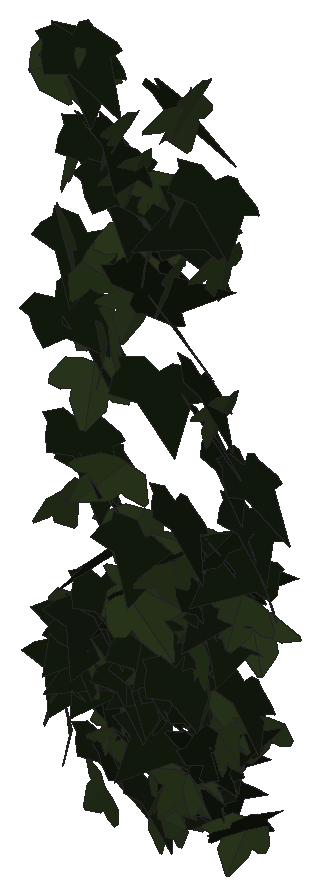
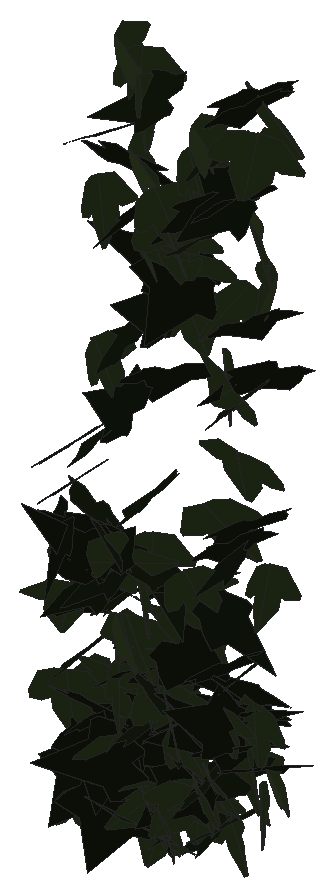
# SketchUp Ruby script. Lengths in inches.
U = 1.inch
M = Sketchup.active_model
def pt(a) = Geom::Point3d.new(a.map { |v| v * U })
def face(e, loops, mat)
  f = e.add_face(loops[0].map { |a| pt(a) })
  loops[1..].each { |l| e.add_face(l.map { |a| pt(a) }).erase! }
  f.material = f.back_material = mat if mat
  f
end
# faces: each face lists its corners as indices into pts; further lists are holes
def faces(e, pts, list, mat = nil) = list.each { |f| face(e, (f[0].is_a?(Array) ? f : [f]).map { |l| l.map { |i| pts[i] } }, mat) }
# xy, xz, yz: faces in a plane at the given z, y or x. An outline is a flat list of corners, or four numbers for a rectangle; further outlines are holes
def ring(l) = l.size == 4 ? [[l[0], l[1]], [l[2], l[1]], [l[2], l[3]], [l[0], l[3]]] : l.each_slice(2).to_a
def flat(e, list, mat, &to3) = list.each { |f| face(e, (f[0].is_a?(Array) ? f : [f]).map { |l| ring(l).map { |u, v| to3.(u, v) } }, mat) }
def xy(e, z, list, mat = nil) = flat(e, list, mat) { |x, y| [x, y, z] }
def xz(e, y, list, mat = nil) = flat(e, list, mat) { |x, z| [x, y, z] }
def yz(e, x, list, mat = nil) = flat(e, list, mat) { |y, z| [x, y, z] }
def lines(e, pts, list) = list.each { |a, b| e.add_line(pt(pts[a]), pt(pts[b])) }
# prism: a flat outline (further loops are holes) pulled along v
def prism(e, loops, v, mat = nil)
  f = face(e, loops, mat); d = Geom::Vector3d.new(v.map { |x| x * U })
  f.pushpull(f.normal.samedirection?(d) ? d.length : -d.length)
end
def box(e, o, s, mat = nil) = prism(e, [[o, [o[0] + s[0], o[1], o[2]], [o[0] + s[0], o[1] + s[1], o[2]], [o[0], o[1] + s[1], o[2]]]], [0, 0, s[2]], mat)
def at(x, y, z, deg = 0) = Geom::Transformation.translation(pt([x, y, z])) * Geom::Transformation.rotation(ORIGIN, Z_AXIS, deg.degrees)
def axes(o, x, y, z) = Geom::Transformation.new([*x, 0, *y, 0, *z, 0, *pt(o).to_a, 1])
def part(name) = M.definitions.add(name)
# library, detail: a bought-in or finely detailed component or shape, given as its bounding box
def library(name, o, s) = part(name).tap { |d| box(d.entities, o, s) }
def detail(e, o, s) = box(e.add_group.entities, o, s)
def put(e, d, t, mat = nil) = e.add_instance(d, t).tap { |i| i.material = mat if mat }
def group(e, t, mat = nil) = e.add_group.tap { |g| g.transformation = t; g.material = mat if mat }.entities
root = M.entities
M.materials.add("1026 AP 7946 SUNNY SIDE UP").color = [254, 231, 186]
M.materials.add("efeu1").color = [18, 25, 13]
M.materials.add("efeu2").color = [43, 57, 29]
c1 = part("ivyleaf_10")
p = [[0,0.5,-0.03],[-0.0625,2.02,-0.43],[-0.19,2.01,-0.46],[-0.54,1.05,-0.29],[-0.52,0.625,-0.18],[-0.83,0.76,-0.28],
  [-1.16,0.64,-0.33],[-1.15,0.33,-0.24],[-0.77,-0.39,0.02],[-0.3,-0.51,0.16],[0.04,-0.48,0.23],[-0.02,2.01,-0.4375],
  [-0.06,2.01,-0.43],[0.04,-0.49,0.23],[0.67,-0.49,0.14],[1.38,0.36,-0.2],[1.375,0.51,-0.24],[0.81,0.65,-0.19],
  [0.62,0.59,-0.15],[0.6,1.09,-0.28],[0.5,1.23,-0.31]]
faces(c1.entities,p,[[0,1,2,3,4,5,6,7,8,9,10],[11,12,0,13,14,15,16,17,18,19,20]],"efeu2")
c2 = part("ivyleaf_9")
p = [[1.54,2.16,1.25],[1.36,2.04,1.19],[-0.21,0.99,0.68],[-0.71,1.11,0.82],[-0.85,0.86,0.67],[-0.8,0.17,0.21],
  [-0.9,-0.01,0.1],[-0.67,-0.16,-0.02],[-0.08,-0.08,-0.05],[-0.03,-0.6,-0.4],[0.65,-0.88,-0.66],[0.83,-0.6,-0.49],
  [1.29,-0.42,-0.43],[1.8125,-0.07,-0.26],[1.21,0.44,0.15]]
faces(c2.entities,p,[[0,1,2,3,4,5,6,7,8,9,10,11,12,13,14]],"efeu1")
put(root,c1,axes([125.9,212.72,288.875],[0.27031,-0.30835,-0.02636],[-0.00295,0.02623,-0.36336],[0.48629,0.17156,0.01245]),"1026 AP 7946 SUNNY SIDE UP")
put(root,c1,axes([125.88,212.42,280.78],[0.18915,-0.27946,0.07883],[0.04242,-0.07342,-0.31384],[0.45429,0.12321,-0.00352]),"1026 AP 7946 SUNNY SIDE UP")
put(root,c1,axes([125.91,212.75,290.12],[-0.49029,-0.16213,-0.04358],[0.07501,-0.00225,-0.36123],[0.25219,-0.31453,0.02272]),"1026 AP 7946 SUNNY SIDE UP")
put(root,c1,axes([125.86,212.73,281.77],[0.4363,-0.17051,-0.03418],[0.03314,0.09342,-0.32184],[0.27083,0.26325,0.09445]),"1026 AP 7946 SUNNY SIDE UP")
put(root,c1,axes([125.91,212.43,283.64],[-0.11924,-0.2929,-0.13998],[0.08747,0.12391,-0.31023],[0.499,-0.09171,0.02093]),"1026 AP 7946 SUNNY SIDE UP")
put(root,c1,axes([125.6,212.43,290.15],[0.31014,-0.19111,-0.25299],[0.32846,-0.13247,0.2795],[-0.36084,-0.28483,0.03698]),"1026 AP 7946 SUNNY SIDE UP")
put(root,c2,axes([125.93,212.75,280.98],[-0.30569,-0.24857,0.06162],[0.05661,-0.10267,-0.31222],[0.39854,-0.17608,0.09162]),"1026 AP 7946 SUNNY SIDE UP")
put(root,c1,axes([126.25,212.53,280.91],[-0.19821,0.12164,0.30818],[-0.38939,0.16855,-0.17753],[-0.32434,-0.27669,0.0248]),"1026 AP 7946 SUNNY SIDE UP")
put(root,c1,axes([125.98,212.35,287.9375],[-0.27058,0.28491,-0.09651],[0.04338,-0.09437,-0.34254],[-0.47039,-0.17259,0.02392]),"1026 AP 7946 SUNNY SIDE UP")
put(root,c2,axes([126.01,212.8,287.54],[-0.20232,-0.3188,0.03575],[0.0034,-0.0402,-0.35397],[0.50455,-0.12757,0.01672]),"1026 AP 7946 SUNNY SIDE UP")
put(root,c1,axes([126.18,212.21,280.22],[0.12911,-0.18145,-0.26592],[-0.07081,0.25619,-0.19959],[0.48971,0.08488,0.04125]),"1026 AP 7946 SUNNY SIDE UP")
put(root,c2,axes([126.17,212.68,281.64],[-0.35105,-0.22264,0.09145],[-0.02769,-0.10742,-0.31927],[0.3766,-0.21543,0.06177]),"1026 AP 7946 SUNNY SIDE UP")
put(root,c2,axes([125.9375,212.77,284.62],[0.03499,-0.32884,-0.11313],[0.0607,0.10985,-0.33591],[0.54081,0.00894,0.04502]),"1026 AP 7946 SUNNY SIDE UP")
put(root,c2,axes([125.89,212.36,286.68],[0.12891,-0.22324,-0.27152],[0.08477,0.27461,-0.22182],[0.53491,0.01028,0.10059]),"1026 AP 7946 SUNNY SIDE UP")
put(root,c1,axes([126.13,212.74,285.45],[0.55471,-0.02774,0.05101],[0.07311,-0.03924,-0.36298],[0.05156,0.35409,-0.03412]),"1026 AP 7946 SUNNY SIDE UP")
put(root,c2,axes([126.08,212.84,286.34],[0.07413,-0.33284,0.0505],[0.00087,-0.05133,-0.34655],[0.52945,0.04669,-0.0065]),"1026 AP 7946 SUNNY SIDE UP")
put(root,c2,axes([126.16,212.62,290.58],[-0.08016,-0.35944,0.00458],[0.00034,-0.00658,-0.37404],[0.56528,-0.05097,0.00088]),"1026 AP 7946 SUNNY SIDE UP")
put(root,c2,axes([126.2,212.88,284.26],[-0.11359,-0.32153,-0.00731],[0.00034,0.00535,-0.33947],[0.50565,-0.07224,-0.00142]),"1026 AP 7946 SUNNY SIDE UP")
put(root,c2,axes([126.09,212.46,290.75],[0.05375,-0.31546,-0.17041],[0.04786,0.16637,-0.32292],[0.55673,0.01615,0.04421]),"1026 AP 7946 SUNNY SIDE UP")
put(root,c2,axes([126.13,212.76,284.125],[0.3525,-0.23972,-0.11649],[-0.14407,0.06698,-0.3371],[0.39011,0.24135,-0.01924]),"1026 AP 7946 SUNNY SIDE UP")
put(root,c1,axes([126.2,212.42,281.45],[-0.34069,0.13509,-0.19375],[0.16571,-0.17294,-0.25302],[-0.32532,-0.22956,0.07403]),"1026 AP 7946 SUNNY SIDE UP")
put(root,c2,axes([126.22,212.93,281.52],[0.07138,-0.00129,0.32422],[0.35069,0.22449,-0.03088],[-0.34918,0.2252,0.03526]),"1026 AP 7946 SUNNY SIDE UP")
put(root,c2,axes([126.42,212.77,281.08],[-0.31851,-0.23754,0.08271],[0.01533,-0.11223,-0.31217],[0.39466,-0.18735,0.07888]),"1026 AP 7946 SUNNY SIDE UP")
put(root,c2,axes([126.25,212.72,289.22],[-0.01907,-0.35238,-0.04597],[0.0006,0.04263,-0.36298],[0.55812,-0.01209,-0.00118]),"1026 AP 7946 SUNNY SIDE UP")
put(root,c2,axes([126.62,212.67,281.27],[-0.38905,-0.15491,0.14585],[-0.16155,-0.10298,-0.2998],[0.2888,-0.26629,0.02878]),"1026 AP 7946 SUNNY SIDE UP")
put(root,c2,axes([126.35,212.63,281.67],[-0.2732,-0.25599,-0.07802],[0.12245,0.03605,-0.31543],[0.40084,-0.18549,0.04318]),"1026 AP 7946 SUNNY SIDE UP")
put(root,c2,axes([126.2,212.74,289.29],[0.51186,-0.12067,-0.05066],[-0.0863,-0.00897,-0.35661],[0.18539,0.329,-0.02612]),"1026 AP 7946 SUNNY SIDE UP")
put(root,c2,axes([126.64,212.5625,283.01],[-0.20337,0.23142,-0.18939],[0.05782,-0.18793,-0.26954],[-0.46242,-0.12527,0.04959]),"1026 AP 7946 SUNNY SIDE UP")
put(root,c2,axes([126.13,212.58,280.71],[0.20887,-0.26076,0.11855],[0.15681,-0.07811,-0.29757],[0.42084,0.15852,0.05204]),"1026 AP 7946 SUNNY SIDE UP")
put(root,c2,axes([126.5,212.5625,281.96],[-0.44635,-0.14929,-0.08709],[0.13609,0.0146,-0.3292],[0.23217,-0.29558,0.02555]),"1026 AP 7946 SUNNY SIDE UP")
put(root,c2,axes([126.29,212.8125,282.09],[0.07857,-0.32043,0.03112],[0.00011,-0.0324,-0.33425],[0.50636,0.04973,-0.00475]),"1026 AP 7946 SUNNY SIDE UP")
put(root,c1,axes([126.5,212.82,281.64],[0.48968,-0.07394,-0.03517],[-0.05512,-0.00175,-0.3296],[0.11529,0.31324,-0.00821]),"1026 AP 7946 SUNNY SIDE UP")
put(root,c2,axes([126.37,212.72,282.35],[0.03697,-0.30768,-0.09831],[0.0408,0.09544,-0.31565],[0.50408,0.01484,0.03276]),"1026 AP 7946 SUNNY SIDE UP")
put(root,c2,axes([126.38,212.71,279.98],[0.08932,-0.30861,-0.02061],[0.0869,0.0284,-0.31726],[0.47828,0.05248,0.06149]),"1026 AP 7946 SUNNY SIDE UP")
put(root,c1,axes([126.78,212.48,284.31],[0.39586,0.12783,-0.19321],[-0.30675,-0.02334,-0.2852],[-0.18425,0.3135,0.0597]),"1026 AP 7946 SUNNY SIDE UP")
put(root,c1,axes([126.52,212.24,287.49],[-0.09273,-0.24523,-0.26318],[0.24366,0.21349,-0.24808],[0.49892,-0.14984,0.07225]),"1026 AP 7946 SUNNY SIDE UP")
put(root,c1,axes([126.34,212.68,286.35],[0.39385,-0.05844,0.25761],[0.36023,-0.10799,-0.26268],[0.18356,0.3373,-0.03723]),"1026 AP 7946 SUNNY SIDE UP")
put(root,c1,axes([126.92,212.05,279.6],[-0.30668,0.14917,0.22949],[-0.33738,0.07661,-0.24687],[-0.25091,-0.28534,0.05145]),"1026 AP 7946 SUNNY SIDE UP")
put(root,c1,axes([126.625,212.65,280.45],[0.35829,-0.19594,0.09833],[0.08114,-0.08731,-0.30845],[0.33375,0.23157,-0.03057]),"1026 AP 7946 SUNNY SIDE UP")
put(root,c1,axes([126.8,212.17,286.36],[0.20652,-0.26363,-0.20979],[-0.04754,0.20698,-0.29712],[0.5202,0.12358,0.05613]),"1026 AP 7946 SUNNY SIDE UP")
put(root,c2,axes([126.45,212.47,281.18],[0.29811,0.09709,0.24138],[0.34076,0.08864,-0.21848],[-0.20564,0.28762,-0.01212]),"1026 AP 7946 SUNNY SIDE UP")
put(root,c1,axes([126.73,212.81,280.33],[0.3077,-0.24861,0.03727],[0.04569,-0.02495,-0.32599],[0.3927,0.1977,0.00872]),"1026 AP 7946 SUNNY SIDE UP")
put(root,c1,axes([126.86,212.87,283.4375],[-0.27049,-0.24659,0.13294],[-0.00508,-0.15148,-0.30028],[0.43863,-0.15382,0.07851]),"1026 AP 7946 SUNNY SIDE UP")
put(root,c2,axes([126.59,212.62,279.84],[0.26914,-0.26132,-0.04178],[-0.04522,0.02786,-0.32153],[0.41301,0.17334,-0.00797]),"1026 AP 7946 SUNNY SIDE UP")
put(root,c1,axes([126.95,212.65,280.22],[-0.41449,-0.18507,0.01137],[0.00557,-0.02604,-0.33109],[0.29157,-0.26259,0.0225]),"1026 AP 7946 SUNNY SIDE UP")
put(root,c2,axes([126.67,212.51,288.95],[0.11307,-0.22963,-0.27403],[0.02992,0.27237,-0.2365],[0.55018,0.03238,0.06918]),"1026 AP 7946 SUNNY SIDE UP")
put(root,c2,axes([126.67,212.73,280.51],[0.19701,-0.29561,0.00896],[0.00684,-0.00942,-0.33081],[0.46505,0.12537,0.00107]),"1026 AP 7946 SUNNY SIDE UP")
put(root,c2,axes([127.07,212.78,282.39],[-0.0711,0.15814,-0.28677],[0.04928,-0.27849,-0.16933],[-0.50222,-0.04971,0.02398]),"1026 AP 7946 SUNNY SIDE UP")
put(root,c1,axes([126.98,212.48,289.76],[0.07132,-0.32502,0.13566],[0.00688,-0.1341,-0.33859],[0.55246,0.04363,-0.0133]),"1026 AP 7946 SUNNY SIDE UP")
put(root,c1,axes([127.23,212.54,282.59],[-0.39985,0.02202,0.20204],[-0.29352,-0.13008,-0.23522],[0.10009,-0.29353,0.11733]),"1026 AP 7946 SUNNY SIDE UP")
put(root,c2,axes([126.83,212.72,288.43],[-0.08218,-0.30684,0.16377],[0.05503,-0.16638,-0.3165],[0.54187,-0.02964,0.05698]),"1026 AP 7946 SUNNY SIDE UP")
put(root,c1,axes([127.05,212.8,281.08],[-0.12394,-0.27894,0.13465],[0.0106,-0.13806,-0.29656],[0.48533,-0.06822,0.04087]),"1026 AP 7946 SUNNY SIDE UP")
put(root,c2,axes([126.93,212.47,289.38],[-0.10267,-0.25655,0.24066],[0.04118,-0.24211,-0.26615],[0.54558,-0.03001,0.06538]),"1026 AP 7946 SUNNY SIDE UP")
put(root,c2,axes([127.01,212.65,281.26],[-0.12456,-0.30558,-0.05106],[0.04831,0.04135,-0.32437],[0.48393,-0.08278,0.01924]),"1026 AP 7946 SUNNY SIDE UP")
put(root,c1,axes([127.04,212.74,280.15],[-0.35078,-0.16321,-0.15919],[0.21561,0.07202,-0.2836],[0.27874,-0.2611,0.01904]),"1026 AP 7946 SUNNY SIDE UP")
put(root,c1,axes([127.21,212.35,289.25],[-0.06477,-0.36023,-0.00274],[0.01132,-0.00021,-0.37345],[0.56631,-0.04119,0.00715]),"1026 AP 7946 SUNNY SIDE UP")
put(root,c2,axes([127.09,212.7,283.28],[-0.201,-0.30566,0.04261],[0.00852,-0.04886,-0.34073],[0.4853,-0.12574,0.02363]),"1026 AP 7946 SUNNY SIDE UP")
put(root,c1,axes([127.25,212.4375,287.1875],[-0.2232,-0.30509,0.10051],[-0.00382,-0.10755,-0.34465],[0.50448,-0.1358,0.04186]),"1026 AP 7946 SUNNY SIDE UP")
put(root,c1,axes([127.08,212.57,287.96],[0.52468,0.11095,0.0094],[0.03089,-0.03233,-0.36045],[-0.17223,0.33222,-0.03603]),"1026 AP 7946 SUNNY SIDE UP")
put(root,c2,axes([126.99,212.62,280.34],[0.50426,-0.02227,-0.0261],[-0.04234,-0.02522,-0.33016],[0.03169,0.32069,-0.02588]),"1026 AP 7946 SUNNY SIDE UP")
put(root,c1,axes([127.375,212.65,288.32],[-0.51079,-0.08402,0.10248],[-0.12848,-0.07825,-0.34179],[0.16016,-0.33075,0.05266]),"1026 AP 7946 SUNNY SIDE UP")
put(root,c1,axes([127.25,212.8,281.48],[0.14073,-0.30596,-0.05661],[-0.00093,0.05521,-0.32773],[0.48831,0.08828,0.01569]),"1026 AP 7946 SUNNY SIDE UP")
put(root,c2,axes([127.11,212.63,287.72],[0.51596,0.0352,-0.11248],[-0.16844,-0.02599,-0.33984],[-0.06535,0.3449,-0.01208]),"1026 AP 7946 SUNNY SIDE UP")
put(root,c2,axes([127.15,212.8,281.21],[-0.1011,-0.30619,0.07614],[0.00569,-0.07792,-0.32218],[0.4959,-0.06153,0.01922]),"1026 AP 7946 SUNNY SIDE UP")
put(root,c2,axes([127.57,212.76,281.625],[-0.35,0.23567,-0.02127],[-0.00684,-0.03425,-0.33303],[-0.37212,-0.22103,0.02613]),"1026 AP 7946 SUNNY SIDE UP")
put(root,c1,axes([127.41,212.76,281.46],[-0.33834,-0.2305,0.07924],[-0.01901,-0.09416,-0.32063],[0.38226,-0.20869,0.05419]),"1026 AP 7946 SUNNY SIDE UP")
put(root,c2,axes([127.52,212.65,280.92],[-0.38418,0.18598,-0.08726],[0.09009,-0.06609,-0.31622],[-0.30917,-0.25036,0.01628]),"1026 AP 7946 SUNNY SIDE UP")
put(root,c1,axes([127.41,212.79,288.8125],[-0.24704,-0.29268,0.1131],[0.00476,-0.12609,-0.33749],[0.49242,-0.14561,0.06]),"1026 AP 7946 SUNNY SIDE UP")
put(root,c2,axes([127.56,212.76,281.42],[-0.48913,-0.08331,0.04318],[-0.05175,-0.04025,-0.33054],[0.13757,-0.31136,0.02919]),"1026 AP 7946 SUNNY SIDE UP")
put(root,c2,axes([127.23,212.61,279.62],[0.08962,-0.30503,0.04262],[0.02998,-0.04026,-0.3197],[0.48346,0.05904,0.01193]),"1026 AP 7946 SUNNY SIDE UP")
put(root,c2,axes([127.67,212.49,283.23],[-0.03751,0.31967,0.07441],[-0.07471,0.06648,-0.32707],[-0.50925,-0.0333,0.0425]),"1026 AP 7946 SUNNY SIDE UP")
put(root,c1,axes([127.38,212.54,288.19],[0.22506,-0.26703,0.19485],[0.16607,-0.15944,-0.31267],[0.48846,0.17724,0.01653]),"1026 AP 7946 SUNNY SIDE UP")
put(root,c2,axes([127.37,212.5625,281.82],[-0.15335,-0.29472,-0.10509],[0.07123,0.09059,-0.31896],[0.48433,-0.10664,0.01364]),"1026 AP 7946 SUNNY SIDE UP")
put(root,c1,axes([127.1875,212.37,282.39],[0.40212,0.09619,0.21799],[0.31879,0.05989,-0.28085],[-0.17714,0.32613,-0.01058]),"1026 AP 7946 SUNNY SIDE UP")
put(root,c1,axes([127.54,212.52,279.67],[0.15211,-0.29945,-0.02419],[0.02958,0.02888,-0.32285],[0.47117,0.09486,0.02808]),"1026 AP 7946 SUNNY SIDE UP")
put(root,c1,axes([127.59,212.78,279.9],[0.33205,-0.22926,0.02963],[0.02797,-0.02449,-0.32123],[0.3625,0.2119,-0.00236]),"1026 AP 7946 SUNNY SIDE UP")
put(root,c2,axes([127.79,212.375,280.69],[-0.47677,-0.08932,-0.02117],[0.04869,-0.03482,-0.32295],[0.13546,-0.30187,0.04157]),"1026 AP 7946 SUNNY SIDE UP")
put(root,c1,axes([127.69,212.53,279.48],[-0.4573,0.1031,-0.00548],[-0.00561,-0.02767,-0.3168],[-0.16228,-0.28957,0.02639]),"1026 AP 7946 SUNNY SIDE UP")
put(root,c2,axes([127.29,212.69,280.9],[0.27655,-0.13567,0.24397],[0.27439,-0.16192,-0.22927],[0.33135,0.24732,-0.01376]),"1026 AP 7946 SUNNY SIDE UP")
put(root,c2,axes([127.79,212.65,282.03],[-0.4428,-0.16436,0.00471],[0.06556,-0.08193,-0.32281],[0.25014,-0.26948,0.09296]),"1026 AP 7946 SUNNY SIDE UP")
put(root,c1,axes([127.72,212.4375,281.57],[-0.36836,-0.20665,-0.07817],[0.11535,0.02939,-0.32055],[0.3257,-0.24413,0.02512]),"1026 AP 7946 SUNNY SIDE UP")
put(root,c2,axes([127.58,212.41,286.1],[-0.14717,-0.32488,-0.10396],[0.09252,0.08569,-0.34629],[0.52599,-0.10598,0.03182]),"1026 AP 7946 SUNNY SIDE UP")
put(root,c2,axes([127.43,212.71,290.27],[0.38875,-0.25535,0.00493],[0.07335,0.03661,-0.36087],[0.39488,0.24458,0.06218]),"1026 AP 7946 SUNNY SIDE UP")
put(root,c1,axes([127.63,212.65,279.9],[-0.21404,-0.15208,-0.24654],[0.289,0.15356,-0.20809],[0.33799,-0.22761,0.0218]),"1026 AP 7946 SUNNY SIDE UP")
put(root,c1,axes([127.85,212.59,290.21],[0.05717,-0.34152,-0.1292],[0.00365,0.12431,-0.35277],[0.57101,0.0334,0.01519]),"1026 AP 7946 SUNNY SIDE UP")
put(root,c1,axes([128.18,212.92,283.32],[-0.08583,-0.03269,-0.32868],[-0.48774,-0.07612,0.0623],[-0.127,0.31442,-0.01712]),"1026 AP 7946 SUNNY SIDE UP")
put(root,c2,axes([127.47,212.5625,287.04],[0.30533,-0.25575,0.15452],[0.11449,-0.13446,-0.33088],[0.45312,0.20631,-0.02052]),"1026 AP 7946 SUNNY SIDE UP")
put(root,c1,axes([127.84,212.65,283],[0.23755,-0.2816,-0.08368],[-0.0022,0.08892,-0.32615],[0.46014,0.1458,0.04164]),"1026 AP 7946 SUNNY SIDE UP")
put(root,c1,axes([127.9,212.72,282.34],[0.48608,-0.0229,-0.11875],[-0.15908,0.11254,-0.30223],[0.09364,0.31008,0.10298]),"1026 AP 7946 SUNNY SIDE UP")
put(root,c1,axes([127.57,212.4375,279.28],[0.01617,-0.14097,-0.29111],[0.28155,-0.22936,0.1236],[-0.40764,-0.16401,0.07382]),"1026 AP 7946 SUNNY SIDE UP")
put(root,c2,axes([127.4,212.1875,287.41],[0.08275,0.01366,0.37283],[0.54351,-0.1108,-0.04813],[0.16958,0.34844,-0.02768]),"1026 AP 7946 SUNNY SIDE UP")
put(root,c2,axes([127.6,212.7,281.11],[0.27487,-0.26612,-0.07423],[-0.01041,0.07948,-0.3253],[0.43277,0.17093,0.03932]),"1026 AP 7946 SUNNY SIDE UP")
put(root,c1,axes([127.88,212.43,287.84],[0.17423,-0.29162,0.15032],[0.05977,-0.14326,-0.3219],[0.51042,0.11632,-0.01362]),"1026 AP 7946 SUNNY SIDE UP")
put(root,c2,axes([128.11,212.41,279.91],[0.24042,0.07623,-0.27791],[-0.37015,-0.13284,-0.17662],[-0.24054,0.2806,-0.00599]),"1026 AP 7946 SUNNY SIDE UP")
put(root,c1,axes([128.17,212.4,279.92],[-0.41834,-0.05121,0.17731],[-0.23948,-0.09959,-0.27318],[0.15042,-0.30098,0.05821]),"1026 AP 7946 SUNNY SIDE UP")
put(root,c2,axes([128.3125,212.71,279.6],[-0.35202,0.20362,0.08688],[-0.2301,-0.04927,-0.28178],[-0.25821,-0.23369,0.13265]),"1026 AP 7946 SUNNY SIDE UP")
put(root,c1,axes([127.96,212.26,283.31],[-0.2445,-0.29763,-0.07063],[0.07417,0.05069,-0.34515],[0.4739,-0.16149,0.01758]),"1026 AP 7946 SUNNY SIDE UP")
put(root,c1,axes([128.03,212.78,282.3125],[0.0562,-0.32454,0.01613],[-0.01457,-0.01862,-0.33627],[0.51084,0.03517,-0.01136]),"1026 AP 7946 SUNNY SIDE UP")
put(root,c2,axes([127.77,212.47,288.62],[0.21967,-0.28443,-0.21016],[-0.0735,0.20079,-0.32277],[0.54397,0.14199,0.04126]),"1026 AP 7946 SUNNY SIDE UP")
put(root,c1,axes([128,212.51,289.14],[0.1664,-0.28543,0.18597],[0.10073,-0.17051,-0.31461],[0.52279,0.1237,0.00142]),"1026 AP 7946 SUNNY SIDE UP")
put(root,c2,axes([127.83,212.47,284.17],[0.13057,-0.3365,0.0424],[0.00337,-0.04382,-0.35722],[0.53343,0.08265,-0.00813]),"1026 AP 7946 SUNNY SIDE UP")
put(root,c1,axes([128.11,212.28,290.4],[-0.21079,-0.33579,-0.08193],[0.05965,0.0684,-0.37194],[0.53862,-0.13899,0.00913]),"1026 AP 7946 SUNNY SIDE UP")
put(root,c1,axes([128.14,212.7,281.53],[-0.03997,-0.30709,-0.10978],[0.02578,0.10379,-0.31674],[0.50956,-0.02934,0.00741]),"1026 AP 7946 SUNNY SIDE UP")
put(root,c1,axes([128.18,212.46,282.02],[0.36393,-0.1934,-0.13732],[-0.10735,0.12209,-0.30642],[0.35238,0.23694,0.04847]),"1026 AP 7946 SUNNY SIDE UP")
put(root,c2,axes([127.97,212.66,281.68],[-0.04519,-0.32011,-0.01295],[0.03745,0.00863,-0.3302],[0.50222,-0.02945,0.02346]),"1026 AP 7946 SUNNY SIDE UP")
put(root,c2,axes([128.11,212.86,279.74],[0.32306,0.23548,-0.03305],[-0.0083,-0.03964,-0.32138],[-0.37389,0.20435,-0.02142]),"1026 AP 7946 SUNNY SIDE UP")
put(root,c2,axes([127.96,212.65,282.9],[0.21519,-0.29114,-0.05409],[-0.02796,0.04782,-0.33111],[0.46388,0.13794,0.00513]),"1026 AP 7946 SUNNY SIDE UP")
put(root,c2,axes([127.99,212.29,281.74],[0.03264,-0.31068,-0.11091],[0.03688,0.10724,-0.31876],[0.51479,0.01202,0.02987]),"1026 AP 7946 SUNNY SIDE UP")
put(root,c1,axes([128.23,212.48,290.68],[0.12379,-0.31932,0.16777],[0.0303,-0.16458,-0.33924],[0.56411,0.07891,-0.01859]),"1026 AP 7946 SUNNY SIDE UP")
put(root,c2,axes([128.01,212.89,283.3],[0.40207,-0.17857,-0.0971],[-0.09588,0.07499,-0.31979],[0.30189,0.26164,0.02776]),"1026 AP 7946 SUNNY SIDE UP")
put(root,c2,axes([127.97,212.76,280.36],[0.27619,0.08911,0.30268],[0.38754,0.15994,-0.20118],[-0.28659,0.30215,0.01964]),"1026 AP 7946 SUNNY SIDE UP")
put(root,c2,axes([127.94,212.77,285.52],[0.23261,-0.2586,0.19521],[0.11658,-0.17709,-0.30728],[0.49184,0.16428,-0.01949]),"1026 AP 7946 SUNNY SIDE UP")
put(root,c1,axes([128.23,212.85,280.59],[0.07469,0.31122,0.04713],[-0.00068,0.04455,-0.32398],[-0.49422,0.04697,0.00757]),"1026 AP 7946 SUNNY SIDE UP")
put(root,c2,axes([128.61,212.32,288.9375],[-0.55107,-0.00514,0.0516],[-0.07722,-0.04369,-0.35867],[0.01766,-0.35132,0.04177]),"1026 AP 7946 SUNNY SIDE UP")
put(root,c1,axes([128.26,212.41,280.03],[0.04566,0.29451,0.12671],[0.00597,0.1215,-0.30406],[-0.50081,0.0283,0.00793]),"1026 AP 7946 SUNNY SIDE UP")
put(root,c2,axes([128.14,212.92,283.28],[-0.06256,-0.10102,0.31499],[0.17211,-0.29457,-0.08715],[0.4771,0.09302,0.07274]),"1026 AP 7946 SUNNY SIDE UP")
put(root,c2,axes([128.53,212.14,280.74],[0.30289,0.04258,-0.26702],[-0.39674,-0.06042,-0.20357],[-0.11615,0.31743,-0.00098]),"1026 AP 7946 SUNNY SIDE UP")
put(root,c1,axes([128.5,212.28,281.49],[0.14634,-0.25897,-0.1993],[-0.0192,0.19686,-0.27849],[0.50653,0.08228,0.04702]),"1026 AP 7946 SUNNY SIDE UP")
put(root,c2,axes([128.53,212.71,282.9],[-0.47181,-0.08346,-0.10979],[0.20238,-0.09892,-0.29541],[0.06398,-0.3025,0.1248]),"1026 AP 7946 SUNNY SIDE UP")
put(root,c2,axes([128.72,212.47,283.76],[-0.07373,0.28715,0.16039],[-0.09725,0.14498,-0.29692],[-0.50308,-0.07011,0.03389]),"1026 AP 7946 SUNNY SIDE UP")
put(root,c2,axes([128.53,212.57,280.4],[0.17926,0.29231,-0.0291],[0.00123,-0.03238,-0.32316],[-0.46202,0.11333,-0.01215]),"1026 AP 7946 SUNNY SIDE UP")
put(root,c2,axes([128.27,212.48,286.25],[0.15469,-0.30172,0.13571],[0.06242,-0.12742,-0.32768],[0.515,0.10608,-0.00105]),"1026 AP 7946 SUNNY SIDE UP")
put(root,c2,axes([128.3,212.85,283],[0.44761,-0.1457,-0.05667],[-0.0598,0.04433,-0.32841],[0.23699,0.28637,0.02416]),"1026 AP 7946 SUNNY SIDE UP")
put(root,c2,axes([128.4,212.77,280.95],[0.00613,-0.32209,-0.01742],[-0.00527,0.01504,-0.33173],[0.50698,0.00405,-0.00324]),"1026 AP 7946 SUNNY SIDE UP")
put(root,c2,axes([128.39,212.86,284.99],[0.07977,-0.31616,0.0957],[-0.00304,-0.09609,-0.33],[0.51895,0.04804,-0.01665]),"1026 AP 7946 SUNNY SIDE UP")
put(root,c2,axes([128.84,212.78,281.03],[-0.49844,0.00328,0.02085],[-0.0322,-0.05888,-0.32123],[0.00084,-0.31213,0.05893]),"1026 AP 7946 SUNNY SIDE UP")
put(root,c1,axes([128.66,212.45,286.02],[-0.02937,-0.33901,0.05866],[0.0062,-0.05916,-0.35005],[0.541,-0.01772,0.0072]),"1026 AP 7946 SUNNY SIDE UP")
put(root,c1,axes([128.39,212.5,281.24],[-0.28803,0.01568,-0.26836],[0.3473,-0.16039,-0.17083],[-0.21882,-0.2752,0.08211]),"1026 AP 7946 SUNNY SIDE UP")
put(root,c2,axes([128.6,212.75,282.51],[-0.19304,-0.29951,0.05826],[-0.00049,-0.06267,-0.33299],[0.47978,-0.12058,0.0231]),"1026 AP 7946 SUNNY SIDE UP")
put(root,c2,axes([128.5,212.47,289.35],[-0.09162,-0.34857,0.02069],[0.10609,-0.03318,-0.35666],[0.53884,-0.05273,0.07374]),"1026 AP 7946 SUNNY SIDE UP")
put(root,c1,axes([128.75,212.33,288.32],[-0.08701,-0.34822,-0.05414],[0.03026,0.04812,-0.36276],[0.55245,-0.05748,0.01135]),"1026 AP 7946 SUNNY SIDE UP")
put(root,c2,axes([128.36,212.88,283.14],[0.05355,-0.02499,0.33328],[0.41576,-0.18665,-0.0446],[0.2961,0.2666,0.00235]),"1026 AP 7946 SUNNY SIDE UP")
put(root,c2,axes([128.95,212.74,283.59],[-0.50022,-0.10011,0.0163],[-0.00974,-0.03468,-0.34227],[0.15921,-0.31666,0.03027]),"1026 AP 7946 SUNNY SIDE UP")
put(root,c1,axes([128.96,212.48,283],[-0.51279,0.03724,0.05577],[-0.10073,-0.12345,-0.31201],[-0.02172,-0.30663,0.13028]),"1026 AP 7946 SUNNY SIDE UP")
put(root,c1,axes([128.88,212.64,279.46],[-0.26977,-0.22945,0.14203],[0.04788,-0.18076,-0.2694],[0.41924,-0.127,0.12216]),"1026 AP 7946 SUNNY SIDE UP")
put(root,c1,axes([129.05,212.68,281.125],[-0.45956,-0.11883,0.05108],[-0.05412,-0.04815,-0.32371],[0.19552,-0.29262,0.03048]),"1026 AP 7946 SUNNY SIDE UP")
put(root,c2,axes([128.7,212.04,280.67],[0.00338,0.02632,0.3489],[0.47512,0.15427,-0.01343],[-0.24354,0.30133,-0.02136]),"1026 AP 7946 SUNNY SIDE UP")
put(root,c2,axes([128.73,212.85,284.87],[0.15742,-0.31059,-0.07307],[0.01644,0.07568,-0.33407],[0.50006,0.09529,0.03399]),"1026 AP 7946 SUNNY SIDE UP")
put(root,c2,axes([128.79,212.74,281.62],[0.05888,-0.31713,0.06602],[0.00047,-0.06629,-0.32927],[0.5093,0.03672,-0.00733]),"1026 AP 7946 SUNNY SIDE UP")
put(root,c1,axes([129,212.09,281.08],[0.00871,0.2678,0.18604],[-0.10617,0.17608,-0.2681],[-0.49529,-0.03303,0.06074]),"1026 AP 7946 SUNNY SIDE UP")
put(root,c2,axes([128.9375,212.3,279.66],[0.23827,0.24983,0.14252],[0.09479,0.12346,-0.30006],[-0.43782,0.16269,0.0126]),"1026 AP 7946 SUNNY SIDE UP")
put(root,c2,axes([128.8125,212.83,284.24],[0.02835,-0.32609,0.02718],[0.0132,-0.02781,-0.33654],[0.51449,0.01868,0.00714]),"1026 AP 7946 SUNNY SIDE UP")
put(root,c1,axes([128.91,212.76,282.55],[0.37745,0.22258,0.04284],[0.03683,0.03401,-0.33692],[-0.35377,0.24102,0.01063]),"1026 AP 7946 SUNNY SIDE UP")
put(root,c2,axes([129.03,212.73,283.51],[0.33867,-0.13997,-0.25504],[-0.36814,0.08728,-0.26101],[0.25193,0.3157,-0.03856]),"1026 AP 7946 SUNNY SIDE UP")
